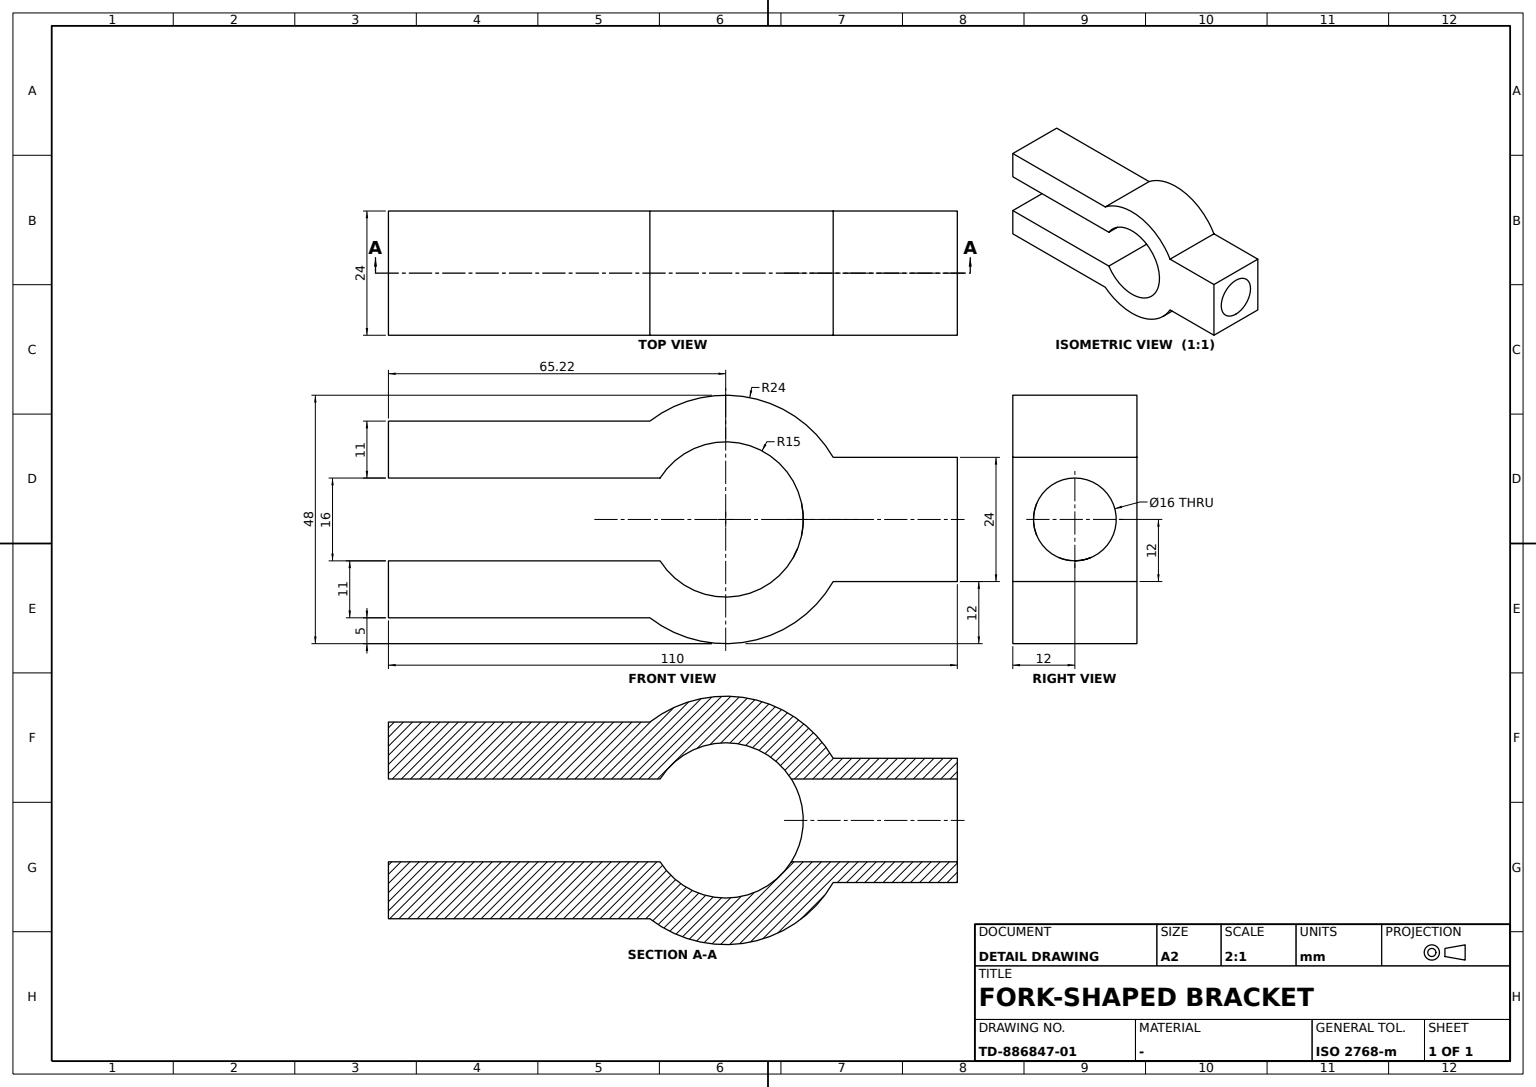
ISO-10303-21;
HEADER;
FILE_DESCRIPTION((''),'2;1');
FILE_NAME('','',(''),(''),'','','');
FILE_SCHEMA(('AUTOMOTIVE_DESIGN'));
ENDSEC;
DATA;
#1=APPLICATION_CONTEXT('');
#2=PRODUCT_CONTEXT('',#1,'mechanical');
#3=PRODUCT('','','',(#2));
#4=PRODUCT_DEFINITION_FORMATION('','',#3);
#5=PRODUCT_DEFINITION_CONTEXT('',#1,'design');
#6=PRODUCT_DEFINITION('','',#4,#5);
#7=PRODUCT_DEFINITION_SHAPE('','',#6);
#8=(LENGTH_UNIT()NAMED_UNIT(*)SI_UNIT(.MILLI.,.METRE.));
#9=(NAMED_UNIT(*)PLANE_ANGLE_UNIT()SI_UNIT($,.RADIAN.));
#10=(NAMED_UNIT(*)SI_UNIT($,.STERADIAN.)SOLID_ANGLE_UNIT());
#11=UNCERTAINTY_MEASURE_WITH_UNIT(LENGTH_MEASURE(0.005),#8,'distance_accuracy_value','');
#12=(GEOMETRIC_REPRESENTATION_CONTEXT(3)GLOBAL_UNCERTAINTY_ASSIGNED_CONTEXT((#11))GLOBAL_UNIT_ASSIGNED_CONTEXT((#8,#9,#10))REPRESENTATION_CONTEXT('',''));
#13=CARTESIAN_POINT('',(20.78461,-12.,12.));
#14=VERTEX_POINT('',#13);
#15=CARTESIAN_POINT('',(20.78461,12.,12.));
#16=VERTEX_POINT('',#15);
#17=DIRECTION('',(0.,1.,0.));
#18=VECTOR('',#17,1000.);
#19=LINE('',#13,#18);
#20=EDGE_CURVE('',#14,#16,#19,.T.);
#21=ORIENTED_EDGE('',*,*,#20,.T.);
#22=CARTESIAN_POINT('',(-14.662878,12.,19.));
#23=VERTEX_POINT('',#22);
#24=CARTESIAN_POINT('',(0.,12.,0.));
#25=DIRECTION('',(0.,0.,1.));
#26=AXIS2_PLACEMENT_3D('',#24,#17,#25);
#27=CIRCLE('',#26,24.);
#28=EDGE_CURVE('',#23,#16,#27,.T.);
#29=ORIENTED_EDGE('',*,*,#28,.F.);
#30=CARTESIAN_POINT('',(-14.662878,-12.,19.));
#31=VERTEX_POINT('',#30);
#32=LINE('',#30,#18);
#33=EDGE_CURVE('',#31,#23,#32,.T.);
#34=ORIENTED_EDGE('',*,*,#33,.F.);
#35=CARTESIAN_POINT('',(0.,-12.,0.));
#36=AXIS2_PLACEMENT_3D('',#35,#17,#25);
#37=CIRCLE('',#36,24.);
#38=EDGE_CURVE('',#31,#14,#37,.T.);
#39=ORIENTED_EDGE('',*,*,#38,.T.);
#40=EDGE_LOOP('',(#21,#29,#34,#39));
#41=FACE_BOUND('',#40,.T.);
#42=CARTESIAN_POINT('',(0.,0.,0.));
#43=DIRECTION('',(-1.,0.,0.));
#44=AXIS2_PLACEMENT_3D('',#42,#17,#43);
#45=CYLINDRICAL_SURFACE('',#44,24.);
#46=ADVANCED_FACE('',(#41),#45,.T.);
#47=CARTESIAN_POINT('',(-65.21539,-12.,-8.));
#48=VERTEX_POINT('',#47);
#49=CARTESIAN_POINT('',(-65.21539,12.,-8.));
#50=VERTEX_POINT('',#49);
#51=CARTESIAN_POINT('',(-65.21539,0.,-8.));
#52=LINE('',#51,#18);
#53=EDGE_CURVE('',#48,#50,#52,.T.);
#54=ORIENTED_EDGE('',*,*,#53,.F.);
#55=CARTESIAN_POINT('',(-12.688578,-12.,-8.));
#56=VERTEX_POINT('',#55);
#57=CARTESIAN_POINT('',(0.,-12.,-8.));
#58=DIRECTION('',(1.,0.,0.));
#59=VECTOR('',#58,1000.);
#60=LINE('',#57,#59);
#61=EDGE_CURVE('',#48,#56,#60,.T.);
#62=ORIENTED_EDGE('',*,*,#61,.T.);
#63=CARTESIAN_POINT('',(-12.688578,12.,-8.));
#64=VERTEX_POINT('',#63);
#65=LINE('',#55,#18);
#66=EDGE_CURVE('',#56,#64,#65,.T.);
#67=ORIENTED_EDGE('',*,*,#66,.T.);
#68=CARTESIAN_POINT('',(0.,12.,-8.));
#69=LINE('',#68,#59);
#70=EDGE_CURVE('',#50,#64,#69,.T.);
#71=ORIENTED_EDGE('',*,*,#70,.F.);
#72=EDGE_LOOP('',(#54,#62,#67,#71));
#73=FACE_BOUND('',#72,.T.);
#74=AXIS2_PLACEMENT_3D('',#51,#25,#58);
#75=PLANE('',#74);
#76=ADVANCED_FACE('',(#73),#75,.T.);
#77=CARTESIAN_POINT('',(-12.688578,12.,8.));
#78=VERTEX_POINT('',#77);
#79=CIRCLE('',#26,15.);
#80=EDGE_CURVE('',#78,#64,#79,.T.);
#81=ORIENTED_EDGE('',*,*,#80,.T.);
#82=ORIENTED_EDGE('',*,*,#66,.F.);
#83=CARTESIAN_POINT('',(-12.688578,-12.,8.));
#84=VERTEX_POINT('',#83);
#85=CIRCLE('',#36,15.);
#86=EDGE_CURVE('',#84,#56,#85,.T.);
#87=ORIENTED_EDGE('',*,*,#86,.F.);
#88=LINE('',#83,#18);
#89=EDGE_CURVE('',#84,#78,#88,.T.);
#90=ORIENTED_EDGE('',*,*,#89,.T.);
#91=EDGE_LOOP('',(#81,#82,#87,#90));
#92=FACE_BOUND('',#91,.T.);
#93=CARTESIAN_POINT('',(15.,-8.,0.));
#94=VERTEX_POINT('',#93);
#95=CARTESIAN_POINT('',(14.756002,-7.554868,3.214669));
#96=CARTESIAN_POINT('',(15.121346,-8.221358,-0.004026));
#97=CARTESIAN_POINT('',(14.758615,-7.559699,-3.198565));
#98=CARTESIAN_POINT('',(13.901161,-5.789473,-5.801999));
#99=CARTESIAN_POINT('',(12.984017,-3.205384,-7.552706));
#100=CARTESIAN_POINT('',(12.543028,-0.029394,-8.21992));
#101=CARTESIAN_POINT('',(12.975467,3.181854,-7.567407));
#102=CARTESIAN_POINT('',(13.89626,5.777271,-5.812409));
#103=CARTESIAN_POINT('',(14.753303,7.549734,-3.224241));
#104=CARTESIAN_POINT('',(15.12133,8.221331,-0.014346));
#105=CARTESIAN_POINT('',(14.761327,7.564852,3.188856));
#106=CARTESIAN_POINT('',(13.903465,5.795026,5.796905));
#107=CARTESIAN_POINT('',(12.984758,3.209136,7.551681));
#108=CARTESIAN_POINT('',(12.542658,0.02942,8.22043));
#109=CARTESIAN_POINT('',(12.976206,-3.185655,7.566392));
#110=CARTESIAN_POINT('',(13.898563,-5.782819,5.807312));
#111=B_SPLINE_CURVE_WITH_KNOTS('',3,(#95,#96,#97,#98,#99,#100,#101,#102,#103,#104,#105,#106,#107,#108,#109,#110,#95,#96,#97),.UNSPECIFIED.,.T.,.F.,(1,1,1,1,1,1,1,1,1,1,1,1,1,1,1,1,1,1,1,1,1,1,1),(-0.009558124,-0.006372082,-0.003186041,0.,0.003186041,0.006372082,0.009558124,0.012744165,0.015930206,0.019116247,0.022302289,0.02548833,0.028674371,0.031860412,0.035046454,0.038232495,0.041418536,0.044604577,0.047790619,0.05097666,0.054162701,0.057348742,0.060534783),.UNSPECIFIED.);
#112=EDGE_CURVE('',#94,#94,#111,.T.);
#113=ORIENTED_EDGE('',*,*,#112,.T.);
#114=EDGE_LOOP('',(#113));
#115=FACE_BOUND('',#114,.T.);
#116=CYLINDRICAL_SURFACE('',#44,15.);
#117=ADVANCED_FACE('',(#92,#115),#116,.F.);
#118=CARTESIAN_POINT('',(44.78461,0.,-8.));
#119=VERTEX_POINT('',#118);
#120=CARTESIAN_POINT('',(44.78461,0.,0.));
#121=DIRECTION('',(0.,0.,-1.));
#122=AXIS2_PLACEMENT_3D('',#120,#58,#121);
#123=CIRCLE('',#122,8.);
#124=EDGE_CURVE('',#119,#119,#123,.T.);
#125=ORIENTED_EDGE('',*,*,#124,.T.);
#126=EDGE_LOOP('',(#125));
#127=FACE_BOUND('',#126,.T.);
#128=ORIENTED_EDGE('',*,*,#112,.F.);
#129=EDGE_LOOP('',(#128));
#130=FACE_BOUND('',#129,.T.);
#131=CARTESIAN_POINT('',(-10.87539,0.,0.));
#132=AXIS2_PLACEMENT_3D('',#131,#58,#17);
#133=CYLINDRICAL_SURFACE('',#132,8.);
#134=ADVANCED_FACE('',(#127,#130),#133,.F.);
#135=CARTESIAN_POINT('',(-65.21539,12.,8.));
#136=VERTEX_POINT('',#135);
#137=CARTESIAN_POINT('',(0.,12.,8.));
#138=LINE('',#137,#59);
#139=EDGE_CURVE('',#136,#78,#138,.T.);
#140=ORIENTED_EDGE('',*,*,#139,.T.);
#141=ORIENTED_EDGE('',*,*,#89,.F.);
#142=CARTESIAN_POINT('',(-65.21539,-12.,8.));
#143=VERTEX_POINT('',#142);
#144=CARTESIAN_POINT('',(0.,-12.,8.));
#145=LINE('',#144,#59);
#146=EDGE_CURVE('',#143,#84,#145,.T.);
#147=ORIENTED_EDGE('',*,*,#146,.F.);
#148=CARTESIAN_POINT('',(-65.21539,0.,8.));
#149=LINE('',#148,#18);
#150=EDGE_CURVE('',#143,#136,#149,.T.);
#151=ORIENTED_EDGE('',*,*,#150,.T.);
#152=EDGE_LOOP('',(#140,#141,#147,#151));
#153=FACE_BOUND('',#152,.T.);
#154=AXIS2_PLACEMENT_3D('',#148,#25,#58);
#155=PLANE('',#154);
#156=ADVANCED_FACE('',(#153),#155,.F.);
#157=CARTESIAN_POINT('',(44.78461,-12.,-12.));
#158=VERTEX_POINT('',#157);
#159=CARTESIAN_POINT('',(20.78461,-12.,-12.));
#160=VERTEX_POINT('',#159);
#161=CARTESIAN_POINT('',(0.,-12.,-12.));
#162=VECTOR('',#43,1000.);
#163=LINE('',#161,#162);
#164=EDGE_CURVE('',#158,#160,#163,.T.);
#165=ORIENTED_EDGE('',*,*,#164,.T.);
#166=CARTESIAN_POINT('',(20.78461,12.,-12.));
#167=VERTEX_POINT('',#166);
#168=LINE('',#159,#18);
#169=EDGE_CURVE('',#160,#167,#168,.T.);
#170=ORIENTED_EDGE('',*,*,#169,.T.);
#171=CARTESIAN_POINT('',(44.78461,12.,-12.));
#172=VERTEX_POINT('',#171);
#173=CARTESIAN_POINT('',(0.,12.,-12.));
#174=LINE('',#173,#162);
#175=EDGE_CURVE('',#172,#167,#174,.T.);
#176=ORIENTED_EDGE('',*,*,#175,.F.);
#177=CARTESIAN_POINT('',(44.78461,0.,-12.));
#178=LINE('',#177,#18);
#179=EDGE_CURVE('',#158,#172,#178,.T.);
#180=ORIENTED_EDGE('',*,*,#179,.F.);
#181=EDGE_LOOP('',(#165,#170,#176,#180));
#182=FACE_BOUND('',#181,.T.);
#183=AXIS2_PLACEMENT_3D('',#177,#121,#43);
#184=PLANE('',#183);
#185=ADVANCED_FACE('',(#182),#184,.T.);
#186=ORIENTED_EDGE('',*,*,#53,.T.);
#187=CARTESIAN_POINT('',(-65.21539,12.,-19.));
#188=VERTEX_POINT('',#187);
#189=CARTESIAN_POINT('',(-65.21539,12.,0.));
#190=VECTOR('',#25,1000.);
#191=LINE('',#189,#190);
#192=EDGE_CURVE('',#188,#50,#191,.T.);
#193=ORIENTED_EDGE('',*,*,#192,.F.);
#194=CARTESIAN_POINT('',(-65.21539,-12.,-19.));
#195=VERTEX_POINT('',#194);
#196=CARTESIAN_POINT('',(-65.21539,0.,-19.));
#197=LINE('',#196,#18);
#198=EDGE_CURVE('',#195,#188,#197,.T.);
#199=ORIENTED_EDGE('',*,*,#198,.F.);
#200=CARTESIAN_POINT('',(-65.21539,-12.,0.));
#201=LINE('',#200,#190);
#202=EDGE_CURVE('',#195,#48,#201,.T.);
#203=ORIENTED_EDGE('',*,*,#202,.T.);
#204=EDGE_LOOP('',(#186,#193,#199,#203));
#205=FACE_BOUND('',#204,.T.);
#206=AXIS2_PLACEMENT_3D('',#196,#43,#25);
#207=PLANE('',#206);
#208=ADVANCED_FACE('',(#205),#207,.T.);
#209=ORIENTED_EDGE('',*,*,#33,.T.);
#210=CARTESIAN_POINT('',(-65.21539,12.,19.));
#211=VERTEX_POINT('',#210);
#212=CARTESIAN_POINT('',(0.,12.,19.));
#213=LINE('',#212,#162);
#214=EDGE_CURVE('',#23,#211,#213,.T.);
#215=ORIENTED_EDGE('',*,*,#214,.T.);
#216=CARTESIAN_POINT('',(-65.21539,-12.,19.));
#217=VERTEX_POINT('',#216);
#218=CARTESIAN_POINT('',(-65.21539,0.,19.));
#219=LINE('',#218,#18);
#220=EDGE_CURVE('',#217,#211,#219,.T.);
#221=ORIENTED_EDGE('',*,*,#220,.F.);
#222=CARTESIAN_POINT('',(0.,-12.,19.));
#223=LINE('',#222,#162);
#224=EDGE_CURVE('',#31,#217,#223,.T.);
#225=ORIENTED_EDGE('',*,*,#224,.F.);
#226=EDGE_LOOP('',(#209,#215,#221,#225));
#227=FACE_BOUND('',#226,.T.);
#228=CARTESIAN_POINT('',(-14.662878,0.,19.));
#229=AXIS2_PLACEMENT_3D('',#228,#121,#43);
#230=PLANE('',#229);
#231=ADVANCED_FACE('',(#227),#230,.F.);
#232=CARTESIAN_POINT('',(44.78461,12.,12.));
#233=VERTEX_POINT('',#232);
#234=CARTESIAN_POINT('',(0.,12.,12.));
#235=LINE('',#234,#162);
#236=EDGE_CURVE('',#233,#16,#235,.T.);
#237=ORIENTED_EDGE('',*,*,#236,.F.);
#238=CARTESIAN_POINT('',(44.78461,12.,0.));
#239=VECTOR('',#121,1000.);
#240=LINE('',#238,#239);
#241=EDGE_CURVE('',#233,#172,#240,.T.);
#242=ORIENTED_EDGE('',*,*,#241,.T.);
#243=ORIENTED_EDGE('',*,*,#175,.T.);
#244=CARTESIAN_POINT('',(-14.662878,12.,-19.));
#245=VERTEX_POINT('',#244);
#246=EDGE_CURVE('',#167,#245,#27,.T.);
#247=ORIENTED_EDGE('',*,*,#246,.T.);
#248=CARTESIAN_POINT('',(0.,12.,-19.));
#249=LINE('',#248,#162);
#250=EDGE_CURVE('',#245,#188,#249,.T.);
#251=ORIENTED_EDGE('',*,*,#250,.T.);
#252=ORIENTED_EDGE('',*,*,#192,.T.);
#253=ORIENTED_EDGE('',*,*,#70,.T.);
#254=ORIENTED_EDGE('',*,*,#80,.F.);
#255=ORIENTED_EDGE('',*,*,#139,.F.);
#256=LINE('',#187,#239);
#257=EDGE_CURVE('',#211,#136,#256,.T.);
#258=ORIENTED_EDGE('',*,*,#257,.F.);
#259=ORIENTED_EDGE('',*,*,#214,.F.);
#260=ORIENTED_EDGE('',*,*,#28,.T.);
#261=EDGE_LOOP('',(#237,#242,#243,#247,#251,#252,#253,#254,#255,#258,#259,#260));
#262=FACE_BOUND('',#261,.T.);
#263=AXIS2_PLACEMENT_3D('',#24,#17,#43);
#264=PLANE('',#263);
#265=ADVANCED_FACE('',(#262),#264,.T.);
#266=ORIENTED_EDGE('',*,*,#124,.F.);
#267=EDGE_LOOP('',(#266));
#268=FACE_BOUND('',#267,.T.);
#269=ORIENTED_EDGE('',*,*,#179,.T.);
#270=ORIENTED_EDGE('',*,*,#241,.F.);
#271=CARTESIAN_POINT('',(44.78461,-12.,12.));
#272=VERTEX_POINT('',#271);
#273=CARTESIAN_POINT('',(44.78461,0.,12.));
#274=LINE('',#273,#18);
#275=EDGE_CURVE('',#272,#233,#274,.T.);
#276=ORIENTED_EDGE('',*,*,#275,.F.);
#277=CARTESIAN_POINT('',(44.78461,-12.,0.));
#278=LINE('',#277,#239);
#279=EDGE_CURVE('',#272,#158,#278,.T.);
#280=ORIENTED_EDGE('',*,*,#279,.T.);
#281=EDGE_LOOP('',(#269,#270,#276,#280));
#282=FACE_BOUND('',#281,.T.);
#283=AXIS2_PLACEMENT_3D('',#273,#58,#121);
#284=PLANE('',#283);
#285=ADVANCED_FACE('',(#268,#282),#284,.T.);
#286=ORIENTED_EDGE('',*,*,#236,.T.);
#287=ORIENTED_EDGE('',*,*,#20,.F.);
#288=CARTESIAN_POINT('',(0.,-12.,12.));
#289=LINE('',#288,#162);
#290=EDGE_CURVE('',#272,#14,#289,.T.);
#291=ORIENTED_EDGE('',*,*,#290,.F.);
#292=ORIENTED_EDGE('',*,*,#275,.T.);
#293=EDGE_LOOP('',(#286,#287,#291,#292));
#294=FACE_BOUND('',#293,.T.);
#295=AXIS2_PLACEMENT_3D('',#273,#121,#43);
#296=PLANE('',#295);
#297=ADVANCED_FACE('',(#294),#296,.F.);
#298=ORIENTED_EDGE('',*,*,#250,.F.);
#299=CARTESIAN_POINT('',(-14.662878,-12.,-19.));
#300=VERTEX_POINT('',#299);
#301=LINE('',#299,#18);
#302=EDGE_CURVE('',#300,#245,#301,.T.);
#303=ORIENTED_EDGE('',*,*,#302,.F.);
#304=CARTESIAN_POINT('',(0.,-12.,-19.));
#305=LINE('',#304,#162);
#306=EDGE_CURVE('',#300,#195,#305,.T.);
#307=ORIENTED_EDGE('',*,*,#306,.T.);
#308=ORIENTED_EDGE('',*,*,#198,.T.);
#309=EDGE_LOOP('',(#298,#303,#307,#308));
#310=FACE_BOUND('',#309,.T.);
#311=CARTESIAN_POINT('',(-14.662878,0.,-19.));
#312=AXIS2_PLACEMENT_3D('',#311,#121,#43);
#313=PLANE('',#312);
#314=ADVANCED_FACE('',(#310),#313,.T.);
#315=ORIENTED_EDGE('',*,*,#61,.F.);
#316=ORIENTED_EDGE('',*,*,#202,.F.);
#317=ORIENTED_EDGE('',*,*,#306,.F.);
#318=EDGE_CURVE('',#160,#300,#37,.T.);
#319=ORIENTED_EDGE('',*,*,#318,.F.);
#320=ORIENTED_EDGE('',*,*,#164,.F.);
#321=ORIENTED_EDGE('',*,*,#279,.F.);
#322=ORIENTED_EDGE('',*,*,#290,.T.);
#323=ORIENTED_EDGE('',*,*,#38,.F.);
#324=ORIENTED_EDGE('',*,*,#224,.T.);
#325=LINE('',#194,#239);
#326=EDGE_CURVE('',#217,#143,#325,.T.);
#327=ORIENTED_EDGE('',*,*,#326,.T.);
#328=ORIENTED_EDGE('',*,*,#146,.T.);
#329=ORIENTED_EDGE('',*,*,#86,.T.);
#330=EDGE_LOOP('',(#315,#316,#317,#319,#320,#321,#322,#323,#324,#327,#328,#329));
#331=FACE_BOUND('',#330,.T.);
#332=AXIS2_PLACEMENT_3D('',#35,#17,#43);
#333=PLANE('',#332);
#334=ADVANCED_FACE('',(#331),#333,.F.);
#335=ORIENTED_EDGE('',*,*,#169,.F.);
#336=ORIENTED_EDGE('',*,*,#318,.T.);
#337=ORIENTED_EDGE('',*,*,#302,.T.);
#338=ORIENTED_EDGE('',*,*,#246,.F.);
#339=EDGE_LOOP('',(#335,#336,#337,#338));
#340=FACE_BOUND('',#339,.T.);
#341=ADVANCED_FACE('',(#340),#45,.T.);
#342=ORIENTED_EDGE('',*,*,#150,.F.);
#343=ORIENTED_EDGE('',*,*,#326,.F.);
#344=ORIENTED_EDGE('',*,*,#220,.T.);
#345=ORIENTED_EDGE('',*,*,#257,.T.);
#346=EDGE_LOOP('',(#342,#343,#344,#345));
#347=FACE_BOUND('',#346,.T.);
#348=ADVANCED_FACE('',(#347),#207,.T.);
#349=CLOSED_SHELL('',(#46,#76,#117,#134,#156,#185,#208,#231,#265,#285,#297,#314,#334,#341,#348));
#350=MANIFOLD_SOLID_BREP('',#349);
#351=ADVANCED_BREP_SHAPE_REPRESENTATION('',(#350),#12);
#352=SHAPE_DEFINITION_REPRESENTATION(#7,#351);
ENDSEC;
END-ISO-10303-21;
